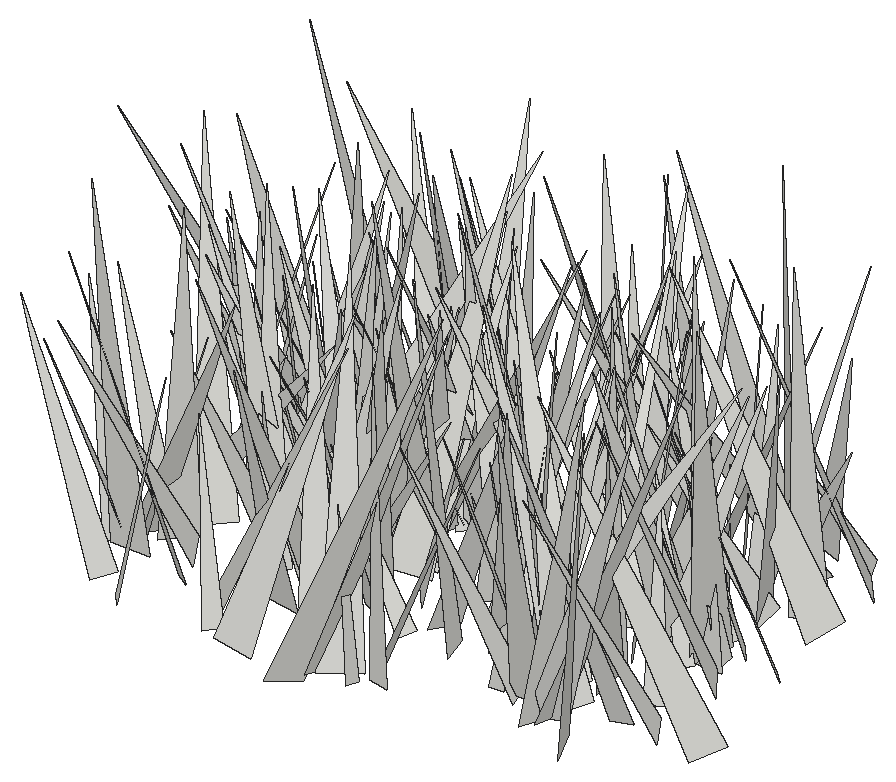
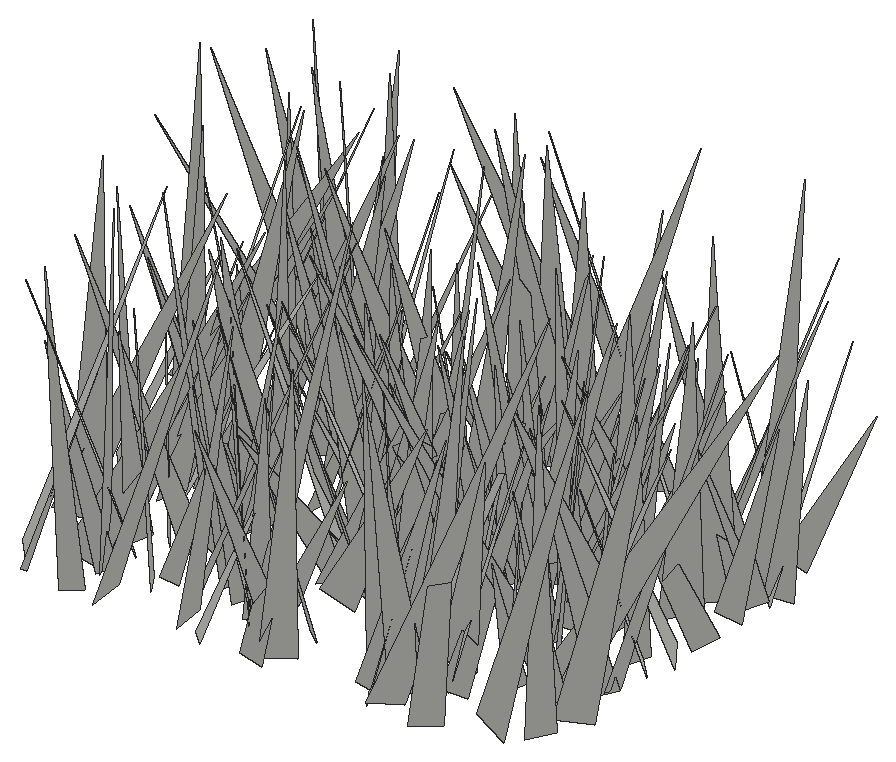
# SketchUp Ruby script. Lengths in inches.
U = 1.inch
M = Sketchup.active_model
def pt(a) = Geom::Point3d.new(a.map { |v| v * U })
def face(e, loops, mat)
  f = e.add_face(loops[0].map { |a| pt(a) })
  loops[1..].each { |l| e.add_face(l.map { |a| pt(a) }).erase! }
  f.material = f.back_material = mat if mat
  f
end
# faces: each face lists its corners as indices into pts; further lists are holes
def faces(e, pts, list, mat = nil) = list.each { |f| face(e, (f[0].is_a?(Array) ? f : [f]).map { |l| l.map { |i| pts[i] } }, mat) }
# xy, xz, yz: faces in a plane at the given z, y or x. An outline is a flat list of corners, or four numbers for a rectangle; further outlines are holes
def ring(l) = l.size == 4 ? [[l[0], l[1]], [l[2], l[1]], [l[2], l[3]], [l[0], l[3]]] : l.each_slice(2).to_a
def flat(e, list, mat, &to3) = list.each { |f| face(e, (f[0].is_a?(Array) ? f : [f]).map { |l| ring(l).map { |u, v| to3.(u, v) } }, mat) }
def xy(e, z, list, mat = nil) = flat(e, list, mat) { |x, y| [x, y, z] }
def xz(e, y, list, mat = nil) = flat(e, list, mat) { |x, z| [x, y, z] }
def yz(e, x, list, mat = nil) = flat(e, list, mat) { |y, z| [x, y, z] }
def lines(e, pts, list) = list.each { |a, b| e.add_line(pt(pts[a]), pt(pts[b])) }
# prism: a flat outline (further loops are holes) pulled along v
def prism(e, loops, v, mat = nil)
  f = face(e, loops, mat); d = Geom::Vector3d.new(v.map { |x| x * U })
  f.pushpull(f.normal.samedirection?(d) ? d.length : -d.length)
end
def box(e, o, s, mat = nil) = prism(e, [[o, [o[0] + s[0], o[1], o[2]], [o[0] + s[0], o[1] + s[1], o[2]], [o[0], o[1] + s[1], o[2]]]], [0, 0, s[2]], mat)
def at(x, y, z, deg = 0) = Geom::Transformation.translation(pt([x, y, z])) * Geom::Transformation.rotation(ORIGIN, Z_AXIS, deg.degrees)
def axes(o, x, y, z) = Geom::Transformation.new([*x, 0, *y, 0, *z, 0, *pt(o).to_a, 1])
def part(name) = M.definitions.add(name)
# library, detail: a bought-in or finely detailed component or shape, given as its bounding box
def library(name, o, s) = part(name).tap { |d| box(d.entities, o, s) }
def detail(e, o, s) = box(e.add_group.entities, o, s)
def put(e, d, t, mat = nil) = e.add_instance(d, t).tap { |i| i.material = mat if mat }
def group(e, t, mat = nil) = e.add_group.tap { |g| g.transformation = t; g.material = mat if mat }.entities
root = M.entities
c1 = part("fur_instance\#9")
p = [[0.8125,0,1.79],[0.67,-0.02,1.48],[0,-0.11,0],[0,0.11,0]]
faces(c1.entities,p,[[0,1,2,3]])
put(root,c1,axes([75.82,233.1,-27.1],[7.81962,-2.04899,1.63917],[-2.46618,-7.49875,2.3913],[-0.8962,2.75717,7.72182]))
put(root,c1,axes([86.82,235.52,-27.1],[6.37942,2.61315,2.43113],[3.05762,-6.56979,-0.96169],[-1.84118,-1.85616,6.82648]))
put(root,c1,axes([67.4,233.97,-27.1],[3.19373,2.97376,0.94617],[2.91746,-3.32577,0.60507],[-1.10768,-0.18543,4.3217]))
put(root,c1,axes([71.48,234.4375,-27.1],[-3.55756,1.9012,0.49829],[1.88183,3.59228,-0.2708],[0.56709,0.00632,4.02461]))
put(root,c1,axes([72.91,233.79,-27.1],[-0.40245,7.17423,1.83924],[7.10701,0.89237,-1.92572],[2.08393,-1.65784,6.92265]))
put(root,c1,axes([70.46,235.91,-27.1],[6.41393,4.45568,0.74677],[4.39818,-5.86174,-2.80093],[1.0328,-2.70854,7.29015]))
put(root,c1,axes([83.7,237.41,-27.1],[0.50064,-7.21064,0.91051],[-7.21991,-0.3887,0.89157],[0.83387,0.96363,7.17281]))
put(root,c1,axes([77.92,234.46,-27.1],[-4.02809,-0.22088,0.67447],[-0.39433,3.92835,-1.06856],[0.59008,1.11738,3.89005]))
put(root,c1,axes([72.41,237.38,-27.1],[-0.34138,-6.1128,0.75859],[-6.1403,0.39794,0.44341],[0.48829,0.7305,6.10625]))
put(root,c1,axes([67.4,238.57,-27.1],[-5.6995,-3.45113,0.56108],[-3.05969,5.44221,2.39374],[1.69215,-1.78365,6.21808]))
put(root,c1,axes([74.41,237.6875,-27.1],[-0.98604,-7.77609,1.14314],[-7.75331,0.77346,-1.42635],[-1.28859,1.29646,7.70749]))
put(root,c1,axes([78.7,234.97,-27.1],[2.01081,5.29668,2.07869],[5.40677,-2.46554,1.0522],[-1.77275,-1.51176,5.56697]))
put(root,c1,axes([64.83,237.87,-27.1],[-3.71629,-3.62879,0.54604],[-3.4741,3.72939,1.13989],[1.18191,-0.44788,5.0675]))
put(root,c1,axes([65.96,235.05,-27.1],[-1.87407,5.07403,0.37598],[4.58214,1.50899,2.47512],[-2.21159,-1.17322,4.80954]))
put(root,c1,axes([83.11,237.68,-27.1],[-5.60277,-1.40853,0.55452],[-1.25772,5.51462,1.29985],[0.84237,-1.13469,5.62898]))
put(root,c1,axes([88.72,238.66,-27.1],[-5.31145,-3.30369,0.30508],[-3.10318,5.15062,1.7494],[1.17379,-1.33255,6.00546]))
put(root,c1,axes([76.02,234.85,-27.1],[-5.00326,5.02156,1.24961],[5.08502,5.09325,-0.10752],[0.95924,-0.80806,7.08781]))
put(root,c1,axes([65.47,237.18,-27.1],[-0.06707,-7.91469,2.47451],[-8.29222,0.04381,-0.08466],[-0.06773,2.47503,7.91452]))
put(root,c1,axes([76.33,234.38,-27.1],[6.99612,0.8962,1.32294],[0.53893,-6.91662,1.83548],[-1.5043,1.69005,6.81028]))
put(root,c1,axes([77.11,234.78,-27.1],[-4.81371,6.17541,1.55135],[6.27572,4.93015,-0.15223],[1.07597,-1.1279,7.82843]))
put(root,c1,axes([68.33,236.62,-27.1],[-4.54723,-4.75664,0.92618],[-4.80738,4.26788,-1.68375],[-0.61038,1.82216,6.36144]))
put(root,c1,axes([85.05,236.82,-27.1],[5.41416,-4.66063,0.97473],[-4.76032,-5.26587,1.26282],[0.1044,1.59183,7.03135]))
put(root,c1,axes([84.84,236.43,-27.1],[6.67765,-1.57713,2.05629],[-1.75682,-6.93326,0.38749],[-1.90506,0.86558,6.85042]))
put(root,c1,axes([81.29,239.26,-27.1],[1.38948,-7.3294,0.52561],[-7.22169,-1.26322,1.47599],[1.35779,0.7818,7.31247]))
put(root,c1,axes([82.22,239.42,-27.1],[-4.28945,-4.51982,0.83876],[-4.25056,4.33652,1.63064],[1.75072,-0.54543,6.01408]))
put(root,c1,axes([74.53,236.67,-27.1],[-0.74897,7.24815,2.93985],[7.55595,1.43371,-1.60981],[2.0214,-2.6736,7.1067]))
put(root,c1,axes([87.3,238.3,-27.1],[-2.01567,-6.30283,1.43527],[-6.28052,1.55369,-1.99742],[-1.52993,1.92587,6.30864]))
put(root,c1,axes([75.15,239.1,-27.1],[-2.33347,-4.94017,0.88075],[-4.99474,2.38012,0.11709],[0.48332,0.74554,5.4623]))
put(root,c1,axes([64.7,237.41,-27.1],[-2.06507,4.56305,1.47225],[4.79287,1.92061,0.77009],[-0.13147,-1.65628,4.94903]))
put(root,c1,axes([85.13,236.9,-27.1],[7.79072,-0.23447,0.87822],[-0.35324,-7.76347,1.06082],[-0.83754,1.09323,7.72172]))
put(root,c1,axes([72.3125,239.3125,-27.1],[-4.28655,1.17606,1.86698],[1.8295,4.17484,1.57066],[1.23356,-2.10497,4.15821]))
put(root,c1,axes([74.13,240.15,-27.1],[5.44226,-5.9088,0.26751],[-5.91243,-5.44486,0.01623],[-0.16928,0.20777,8.03317]))
put(root,c1,axes([91.21,238.4,-27.1],[-4.16636,5.9481,1.52453],[5.74666,3.12806,3.50054],[-2.16332,-3.14611,6.36276]))
put(root,c1,axes([65.1,238.51,-27.1],[5.86888,-2.59714,0.14419],[-2.59865,-5.83866,0.60558],[0.11385,0.61201,6.38922]))
put(root,c1,axes([85.16,240.3125,-27.1],[6.59264,-0.88288,1.14982],[-0.53637,-6.4595,-1.88457],[-1.3468,-1.74924,6.37893]))
put(root,c1,axes([85.06,237.48,-27.1],[-4.32916,0.66549,1.27706],[0.40908,4.44763,-0.93094],[1.38073,0.76884,4.27993]))
put(root,c1,axes([66.33,238.95,-27.1],[-4.86484,4.13925,3.64162],[4.78109,5.5858,0.03796],[2.74517,-2.39309,6.38738]))
put(root,c1,axes([84.28,238.23,-27.1],[-5.98871,-2.33617,1.80164],[-2.60473,6.10133,-0.74665],[1.38529,1.37273,6.38474]))
put(root,c1,axes([77.84,236.35,-27.1],[3.89032,1.8987,0.46131],[1.51623,-3.58179,1.95558],[-1.23244,1.58688,3.86204]))
put(root,c1,axes([85.3125,237.98,-27.1],[-7.32829,2.58062,0.59876],[2.60966,7.33524,0.32553],[0.45582,-0.50666,7.76257]))
put(root,c1,axes([82.47,239.13,-27.1],[5.33637,4.77614,2.80857],[5.34994,-5.45601,-0.88678],[-1.44141,-2.56842,7.10647]))
put(root,c1,axes([79.25,238.71,-27.1],[-6.68963,-2.36331,2.10659],[-2.62997,6.88987,-0.62215],[1.76244,1.31094,7.06748]))
put(root,c1,axes([89.59,239.7,-27.1],[-6.11827,1.22354,0.04324],[1.20265,5.96505,1.37981],[-0.22923,-1.36132,6.08493]))
put(root,c1,axes([77.21,238.49,-27.1],[-1.66623,3.3763,0.05798],[2.90925,1.40249,1.93607],[-1.71436,-0.9015,3.22914]))
put(root,c1,axes([65.49,237.81,-27.1],[3.79033,1.52401,0.8214],[1.29616,-3.80865,1.0854],[-1.14773,0.73179,3.93842]))
put(root,c1,axes([81.27,239.93,-27.1],[-2.39364,-3.13142,1.17859],[-3.27618,2.48779,-0.04385],[0.67935,0.9641,3.94124]))
put(root,c1,axes([68.75,241.16,-27.1],[0.69444,-4.60057,1.02449],[-4.36557,-1.0182,-1.61314],[-1.77671,0.70364,4.36409]))
put(root,c1,axes([82.21,237.4,-27.1],[2.45384,5.3856,0.3895],[5.06414,-2.44383,1.88676],[-1.87372,0.44803,5.60947]))
put(root,c1,axes([83.4375,240.07,-27.1],[-3.37227,-0.8607,0.92289],[-0.91034,3.4828,-0.07828],[0.87397,0.30665,3.4795]))
put(root,c1,axes([88.16,242.69,-27.1],[-5.39374,-4.42373,0.73063],[-4.15874,5.36317,1.77113],[1.67573,-0.92879,6.74722]))
put(root,c1,axes([75.81,241.04,-27.1],[3.73133,2.74864,1.27928],[3.02044,-3.19509,-1.94493],[0.26177,-2.31318,4.20655]))
put(root,c1,axes([65.27,239.65,-27.1],[-1.60239,4.56784,1.22355],[4.62571,1.24567,1.40748],[-0.98238,-1.58525,4.63161]))
put(root,c1,axes([69.11,241.01,-27.1],[3.4639,-0.21189,1.20284],[0.06017,-3.58323,-0.80448],[-1.21988,-0.7784,3.37584]))
put(root,c1,axes([70.13,240.19,-27.1],[-6.35948,3.06032,1.72749],[3.24757,6.48259,0.47123],[1.34279,-1.18457,7.04176]))
put(root,c1,axes([82.43,239.02,-27.1],[3.56611,7.00423,0.23479],[6.50816,-3.2121,-3.02618],[2.59966,-1.56674,7.25387]))
put(root,c1,axes([87.46,240.03,-27.1],[-1.55614,3.71904,0.91385],[3.82438,1.56093,0.15988],[0.20123,-0.90564,4.0283]))
put(root,c1,axes([70.16,240.22,-27.1],[-2.19401,4.08598,0.64459],[3.98986,1.89782,1.55038],[-1.09165,-1.27572,4.37096]))
put(root,c1,axes([73.15,240.28,-27.1],[4.12414,-1.44643,0.07491],[-1.4095,-3.95608,1.21201],[0.33327,1.1677,4.19901]))
put(root,c1,axes([84,239.27,-27.1],[-6.13421,5.52562,0.24546],[5.52788,6.11218,0.5523],[-0.18784,-0.57446,8.23747]))
put(root,c1,axes([70.47,239.15,-27.1],[-6.55915,2.85076,0.80174],[2.70921,6.56329,-1.17278],[1.19574,0.76707,7.05506]))
put(root,c1,axes([82.21,240.03,-27.1],[-0.35457,5.93898,1.63328],[6.05839,0.63143,-0.98081],[1.11129,-1.54746,5.86815]))
put(root,c1,axes([73.56,242.25,-27.1],[-2.21504,-4.22644,0.02495],[-4.06696,2.12371,-1.31133],[-1.15036,0.62998,4.58799]))
put(root,c1,axes([64.6875,241.69,-27.1],[2.58062,-5.27777,0.62862],[-4.46822,-1.77579,3.43383],[2.87837,1.97518,4.76689]))
put(root,c1,axes([69.66,243.11,-27.1],[6.23542,-1.61716,0.46655],[-1.48447,-6.12774,-1.40019],[-0.79324,-1.24458,6.2877]))
put(root,c1,axes([85.625,243.85,-27.1],[5.45366,-4.66647,1.60556],[-4.21255,-5.64853,-2.10822],[-2.57063,-0.64365,6.86103]))
put(root,c1,axes([70.11,241.64,-27.1],[-5.34119,3.3335,0.99515],[3.47843,5.14626,1.43085],[0.05516,-1.74201,6.13133]))
put(root,c1,axes([79.4375,241.07,-27.1],[2.86437,6.58912,2.04567],[6.83224,-2.40073,-1.83379],[0.96006,-2.57407,6.94682]))
put(root,c1,axes([77.86,239.83,-27.1],[7.57177,-0.43303,1.80554],[-0.88332,-7.50835,1.90355],[-1.63317,2.05334,7.34137]))
put(root,c1,axes([81.09,240.08,-27.1],[-3.67286,3.55796,0.5072],[3.52102,3.70767,-0.51167],[0.72023,0.01818,5.08794]))
put(root,c1,axes([74.72,243.12,-27.1],[-1.19832,-8.06423,2.00487],[-8.30399,1.23724,0.01324],[0.30817,1.98109,8.15276]))
put(root,c1,axes([78.06,242.37,-27.1],[3.7544,-3.60472,1.46029],[-3.77286,-3.86843,0.15082],[-0.94444,1.12393,5.20257]))
put(root,c1,axes([84.68,241.25,-27.1],[1.78909,6.44129,2.50482],[6.73985,-2.19865,0.83993],[-1.52927,-2.15428,6.63216]))
put(root,c1,axes([72.03,242.41,-27.1],[-5.02266,3.34128,1.54054],[3.64584,4.87057,1.32283],[0.49523,-1.96924,5.88569]))
put(root,c1,axes([69.45,243.86,-27.1],[3.15853,-4.87453,2.05329],[-4.28659,-3.76007,-2.33247],[-3.09874,0.23284,5.31949]))
put(root,c1,axes([66.7,240.58,-27.1],[-6.24341,4.5177,1.05822],[4.50521,6.32678,-0.4296],[1.11019,-0.26807,7.69449]))
put(root,c1,axes([69.52,242.93,-27.1],[-3.89073,-3.2521,0.98713],[-3.3181,3.95947,-0.03367],[0.73538,0.65937,5.07078]))
put(root,c1,axes([86.81,244.1,-27.1],[7.55718,-3.05255,1.8054],[-2.7949,-7.74218,-1.39129],[-2.18313,-0.65505,8.03077]))
put(root,c1,axes([72.9,242.14,-27.1],[4.30722,-1.10997,0.82887],[-1.21703,-4.32511,0.53238],[-0.66174,0.72977,4.41597]))
put(root,c1,axes([70.14,242.96,-27.1],[-7.66892,-1.90839,0.15613],[-1.91216,7.66661,-0.21311],[0.09999,0.24454,7.89993]))
put(root,c1,axes([66.61,243.5,-27.1],[-5.67591,-0.59927,2.29984],[-0.30227,6.08824,0.84044],[2.35734,-0.66225,5.64524]))
put(root,c1,axes([81.92,242.72,-27.1],[-5.15429,0.32159,0.0951],[0.32057,5.15491,-0.05731],[0.09848,0.05128,5.164]))
put(root,c1,axes([80.93,243.25,-27.1],[-7.3033,-3.33888,1.09507],[-3.45877,7.27632,-0.88176],[0.61989,1.26191,7.98178]))
put(root,c1,axes([69.2,244.77,-27.1],[6.14406,2.36607,3.59044],[3.36505,-6.54408,-1.44586],[-2.67694,-2.79567,6.42319]))
put(root,c1,axes([73.43,245.12,-27.1],[5.23311,-3.59302,0.50013],[-3.53385,-5.24745,-0.7222],[-0.81967,-0.31597,6.30664]))
put(root,c1,axes([71.98,241.91,-27.1],[-5.31881,4.24046,0.31909],[4.24772,5.322,0.07866],[0.20039,-0.26047,6.80184]))
put(root,c1,axes([72.93,240.42,-27.1],[1.87355,6.48838,0.26131],[6.01197,-1.83596,2.48253],[-2.45429,0.45575,6.28063]))
put(root,c1,axes([87.48,244.02,-27.1],[-3.67755,-0.2078,1.11626],[-0.0694,3.8179,0.48208],[1.13331,-0.4405,3.65173]))
put(root,c1,axes([71.16,242.97,-27.1],[1.59622,5.71911,2.00108],[6.0184,-1.73595,0.16062],[-0.70101,-1.88115,5.93551]))
put(root,c1,axes([84.43,242.48,-27.1],[5.20843,4.28763,1.83578],[4.29945,-5.48037,0.60158],[-1.80791,-0.68076,6.71935]))
put(root,c1,axes([89.64,244.41,-27.1],[-3.75562,-3.58045,0.3486],[-3.58145,3.67402,-0.84892],[-0.33818,0.85312,5.11895]))
put(root,c1,axes([65.1875,246.42,-27.1],[-6.16239,-2.08969,1.53365],[-1.42213,6.03269,2.50561],[2.16712,-1.98337,6.00531]))
put(root,c1,axes([79.35,242.23,-27.1],[3.38601,2.0667,0.33408],[1.88033,-3.28152,1.24252],[-0.92044,0.89903,3.76728]))
put(root,c1,axes([86.52,242.93,-27.1],[-0.98772,3.5916,0.11089],[3.35733,0.88143,1.35606],[-1.28071,-0.45933,3.46934]))
put(root,c1,axes([74.43,242.02,-27.1],[-3.17908,7.18759,1.82609],[7.05927,3.54175,-1.65087],[2.27218,-0.9472,7.68392]))
put(root,c1,axes([87.15,243.37,-27.1],[1.25442,7.48082,2.76942],[7.81491,-1.71475,1.09211],[-1.59984,-2.51056,7.50623]))
put(root,c1,axes([72.58,243.89,-27.1],[4.97792,-1.2009,1.19397],[-1.36113,-5.04298,0.6026],[-1.0075,0.87956,5.08515]))
put(root,c1,axes([85.42,243.25,-27.1],[0.44188,5.84269,1.52194],[5.83939,-0.02571,-1.59672],[1.53457,-1.58458,5.63763]))
put(root,c1,axes([74.9,246.1875,-27.1],[1.62052,-5.44249,0.65001],[-5.43307,-1.68456,-0.55967],[-0.72449,0.45919,5.65098]))
put(root,c1,axes([87.62,245.02,-27.1],[-4.41159,-3.54695,0.73212],[-3.61607,4.3782,-0.57829],[0.20221,0.91078,5.63104]))
put(root,c1,axes([73.36,242.16,-27.1],[1.09357,6.43106,0.77169],[6.11568,-1.28298,2.02542],[-2.13365,-0.38127,6.20097]))
put(root,c1,axes([72.23,245.85,-27.1],[-3.11173,-3.4795,0.92655],[-3.33661,3.24675,0.98692],[1.3537,0.0043,4.56244]))
put(root,c1,axes([65.85,244.22,-27.1],[-4.75498,1.70819,1.94206],[1.76287,5.11453,-0.18234],[1.89256,-0.47231,5.04921]))
put(root,c1,axes([73.33,246.44,-27.1],[-3.18461,-4.17271,0.10236],[-4.17132,3.18622,0.10881],[0.1486,0.01532,5.24799]))
put(root,c1,axes([75.9,246.87,-27.1],[-1.54524,-6.7658,0.51217],[-6.71547,1.44992,-1.10738],[-0.96994,0.74015,6.85109]))
put(root,c1,axes([77.31,245.02,-27.1],[6.16664,-2.56617,1.31423],[-2.70082,-6.22755,0.51287],[-1.00896,0.98602,6.65955]))
put(root,c1,axes([69.11,245.34,-27.1],[7.358,-0.55238,1.16955],[-0.51092,-7.44716,-0.30295],[-1.18825,-0.21839,7.37248]))
put(root,c1,axes([73.91,243.53,-27.1],[7.28902,-0.71217,0.57332],[-0.83779,-7.04721,1.89755],[-0.36604,1.94818,7.07364]))
put(root,c1,axes([67.05,247.09,-27.1],[-1.39061,-8.04384,0.83594],[-7.45661,0.94696,-3.29214],[-3.13068,1.31752,7.46987]))
put(root,c1,axes([74.43,242.78,-27.1],[-1.14169,6.19263,0.48775],[6.13199,1.20279,-0.91762],[0.99261,-0.30768,6.22978]))
put(root,c1,axes([67.7,246.54,-27.1],[-3.39488,-3.98848,1.56761],[-3.7052,3.73666,1.48306],[2.15333,0.14147,5.02331]))
put(root,c1,axes([66.82,245.58,-27.1],[-2.76326,-3.0585,1.38467],[-3.15346,2.97986,0.28892],[1.15213,0.82059,4.11176]))
put(root,c1,axes([86.87,243.74,-27.1],[-6.97142,-3.26118,0.0354],[-2.96258,6.29742,-3.28677],[-1.3637,2.99072,6.9594]))
put(root,c1,axes([78.18,246.59,-27.1],[-6.07615,0.58264,0.90457],[0.83184,5.83413,1.82981],[0.68247,-1.92372,5.8233]))
put(root,c1,axes([77.59,244,-27.1],[-3.01404,5.97197,0.86388],[5.95256,2.78442,1.51964],[-0.98886,-1.44144,6.51457]))
put(root,c1,axes([65,243,-27.1],[5.18703,3.91751,0.7095],[3.72248,-5.18551,1.41748],[-1.41191,0.72053,6.34373]))
put(root,c1,axes([74.58,246.28,-27.1],[2.81734,-6.20209,1.85033],[-6.41792,-2.93797,-0.07572],[-0.83667,1.65211,6.81158]))
put(root,c1,axes([77.36,246.38,-27.1],[-4.25466,-1.2014,1.34721],[-0.93808,4.41863,0.97784],[1.54219,-0.62673,4.31153]))
put(root,c1,axes([76.05,245.7,-27.1],[-1.30466,-3.28465,1.2487],[-3.51229,1.2605,-0.354],[0.10971,1.29326,3.5165]))
put(root,c1,axes([77.03,244.09,-27.1],[4.58247,4.01128,0.43645],[4.00699,-4.60163,0.22113],[-0.47421,-0.12046,6.08609]))
put(root,c1,axes([79.41,243.99,-27.1],[-0.73079,4.32054,0.1844],[4.30671,0.74406,-0.36572],[0.39156,-0.12013,4.36662]))
put(root,c1,axes([86.65,247.64,-27.1],[-4.86866,0.51762,1.11395],[0.97098,4.41082,2.19421],[0.75234,-2.34296,4.3769]))
put(root,c1,axes([78.57,245.125,-27.1],[5.68273,3.19615,0.64935],[3.24559,-5.67036,-0.49352],[-0.32122,-0.74969,6.50117]))
put(root,c1,axes([82.98,245.58,-27.1],[2.29321,-4.71361,1.70331],[-4.8602,-1.63403,2.02152],[1.22385,2.34308,4.83635]))
put(root,c1,axes([67.81,243.09,-27.1],[-5.19171,3.73852,1.55221],[3.028,5.26206,-2.54592],[2.68647,1.29382,5.8693]))
put(root,c1,axes([86.6,245.11,-27.1],[-5.80582,1.67481,0.45332],[1.66732,5.82342,-0.1609],[0.48013,0.02943,6.04042]))
put(root,c1,axes([75.09,245.7,-27.1],[-3.69691,-1.68274,0.52652],[-1.75981,3.59718,-0.85985],[0.10916,1.00233,3.96981]))
put(root,c1,axes([65.32,244.39,-27.1],[3.04107,3.48011,0.59696],[3.3547,-3.09349,0.94446],[-1.10161,0.1866,4.52408]))
put(root,c1,axes([65.24,246.77,-27.1],[2.87453,-4.20489,0.68169],[-4.14129,-2.56592,1.63539],[0.99777,1.46412,4.82385]))
put(root,c1,axes([86.32,247.76,-27.1],[6.10646,0.88523,1.50787],[1.27518,-6.00248,-1.64024],[-1.19633,-1.87958,5.94829]))
put(root,c1,axes([82.58,245.01,-27.1],[-5.70861,3.53079,2.01517],[3.32922,6.05385,-1.17592],[2.33318,0.00055,6.60847]))
put(root,c1,axes([68.99,247.32,-27.1],[-4.42725,-2.60663,1.07476],[-2.66002,4.52485,0.01676],[0.93485,0.53053,5.13759]))
put(root,c1,axes([74.09,245.88,-27.1],[-3.60805,2.068,0.36238],[2.05277,3.62596,-0.25393],[0.44056,0.04128,4.15092]))
put(root,c1,axes([66.03,248.58,-27.1],[-3.26059,-4.43586,0.10579],[-4.43536,3.26207,0.0775],[0.12511,0.03932,5.50476]))
put(root,c1,axes([82.9,245.93,-27.1],[-6.0397,-1.24718,1.08354],[-1.47294,5.92489,-1.39057],[0.74831,1.59618,6.00831]))
put(root,c1,axes([69.53,250.18,-27.1],[4.70734,-3.12135,0.14145],[-2.64852,-4.12178,-2.81392],[-1.65776,-2.27815,4.89732]))
put(root,c1,axes([72.9,244.54,-27.1],[-1.71935,6.00909,0.23442],[5.94835,1.73522,-0.85232],[0.8839,0.01135,6.19184]))
put(root,c1,axes([88.93,248.03,-27.1],[-7.28796,2.50197,0.93453],[2.66483,6.99355,2.0583],[0.17855,-2.25345,7.42547]))
put(root,c1,axes([82.76,243.8,-27.1],[-4.41357,6.91206,0.00056],[6.86097,4.38103,-0.99489],[0.83882,0.53496,8.14041]))
put(root,c1,axes([82.66,247.55,-27.1],[-2.78435,-5.66723,3.39056],[-5.97834,3.72634,1.319],[2.80584,2.3158,6.17497]))
put(root,c1,axes([75.77,247.13,-27.1],[4.35224,4.23695,0.82253],[4.28263,-4.09432,-1.57033],[0.53605,-1.68972,5.86752]))
put(root,c1,axes([64.83,249.1,-27.1],[4.91943,-4.73173,2.30235],[-4.40019,-5.42749,-1.75256],[-2.8859,0.2095,6.59686]))
put(root,c1,axes([86.2,250.79,-27.1],[2.18391,-6.70079,0.42323],[-6.08063,-2.16263,-2.86325],[-2.84706,-0.52116,6.43986]))
put(root,c1,axes([84.6,247.8125,-27.1],[2.87799,2.64757,1.74089],[2.94858,-3.09885,-0.16173],[-1.16026,-1.30792,3.90721]))
put(root,c1,axes([80.87,251.1875,-27.1],[-6.78403,-3.28205,0.63683],[-2.89291,6.48484,2.60352],[1.67585,-2.09175,7.07224]))
put(root,c1,axes([87.93,248.39,-27.1],[1.68119,-6.78383,2.85706],[-7.30642,-1.89388,-0.19753],[-0.89411,2.72073,6.98625]))
put(root,c1,axes([83.46,247.74,-27.1],[6.47298,0.85818,0.33872],[0.84258,-6.4766,0.30739],[-0.37587,0.26066,6.52238]))
put(root,c1,axes([67.67,249.43,-27.1],[3.15596,1.30372,1.61225],[1.82364,-3.14251,-1.02861],[-0.98659,-1.6383,3.25603]))
put(root,c1,axes([80.8125,249.11,-27.1],[3.7872,-0.0255,0.26622],[0.02172,-3.73751,-0.66706],[-0.26655,-0.66693,3.72808]))
put(root,c1,axes([70.03,249.9,-27.1],[-3.79874,-3.55526,0.6962],[-3.51199,3.8615,0.55657],[0.88909,0.06302,5.17306]))
put(root,c1,axes([79.05,245.22,-27.1],[-4.90566,2.32822,0.51514],[1.6552,4.17303,-3.098],[1.71648,2.62995,4.45965]))
put(root,c1,axes([68.17,246.625,-27.1],[0.84349,7.5995,0.98427],[7.14395,-0.42161,-2.86687],[2.77222,-1.22577,7.08837]))
put(root,c1,axes([82.73,250.12,-27.1],[0.53786,-3.60504,0.14249],[-3.55289,-0.5543,-0.6129],[-0.62738,0.04841,3.59304]))
put(root,c1,axes([78.45,248.54,-27.1],[-1.80359,3.13263,0.44398],[3.00697,1.53819,1.36218],[-0.98418,-1.04117,3.34825]))
put(root,c1,axes([73.66,248.06,-27.1],[0.00503,4.167,0.7042],[4.17874,-0.11,0.62111],[-0.63075,-0.69557,4.12045]))
put(root,c1,axes([72.98,249.04,-27.1],[4.34542,2.75412,2.00138],[2.98226,-4.64462,-0.0836],[-1.6422,-1.14703,5.14401]))
put(root,c1,axes([77.11,247.42,-27.1],[-1.95645,6.57203,0.15793],[5.85701,1.66776,3.15567],[-2.98529,-1.03499,6.08778]))
put(root,c1,axes([79.6875,249.49,-27.1],[5.0608,-1.8582,0.79428],[-1.91101,-5.09708,0.2516],[-0.65714,0.51221,5.38529]))
put(root,c1,axes([78.59,250.46,-27.1],[4.23217,0.79223,1.75299],[1.35483,-4.23497,-1.35698],[-1.36567,-1.74623,4.08626]))
put(root,c1,axes([69.9375,251.125,-27.1],[-3.5221,-6.63629,1.77015],[-6.5539,3.84233,1.36448],[2.0543,0.8804,7.38808]))
put(root,c1,axes([66.11,248.4,-27.1],[0.58745,4.61701,1.14714],[4.75417,-0.52722,-0.31264],[0.17496,-1.17604,4.64372]))
put(root,c1,axes([88.25,251.58,-27.1],[-5.65228,-5.31186,0.60473],[-5.29476,5.68375,0.43618],[0.73959,0.09466,7.74428]))
put(root,c1,axes([85.47,248.43,-27.1],[-4.49774,2.41965,1.22715],[2.26445,4.65664,-0.88215],[1.49428,0.22634,5.03052]))
put(root,c1,axes([65.13,250.64,-27.1],[5.79339,-2.08626,1.56673],[-1.97661,-6.00002,-0.68061],[-1.70297,-0.13319,6.11985]))
put(root,c1,axes([76.8,252.8,-27.1],[-3.41876,-7.6362,0.72671],[-7.48826,3.49493,1.49637],[1.66304,0.03883,8.23167]))
put(root,c1,axes([84.99,250.88,-27.1],[1.43751,-4.12245,0.23292],[-3.7226,-1.18725,1.96162],[1.78636,0.84328,3.90039]))
put(root,c1,axes([71,252.29,-27.1],[-7.92224,1.63819,2.17065],[2.33717,7.51957,2.85498],[1.39032,-3.306,7.56932]))
put(root,c1,axes([68.85,252.64,-27.1],[6.56004,-2.8558,0.90961],[-2.50702,-6.42798,-2.10074],[-1.6425,-1.59457,6.83935]))
put(root,c1,axes([68.02,248.45,-27.1],[-3.33951,2.40161,0.05247],[2.31618,3.24301,-1.02031],[0.63702,0.79874,3.98485]))
put(root,c1,axes([72.96,250.1,-27.1],[5.47635,-0.94494,2.24683],[-1.1073,-5.8869,0.22307],[-2.17142,0.61884,5.55279]))
put(root,c1,axes([76.0625,250.09,-27.1],[4.67492,4.49227,1.13099],[4.6277,-4.45606,-1.42912],[0.20972,-1.8104,6.324]))
put(root,c1,axes([70.71,248.45,-27.1],[-2.20757,6.36235,0.08993],[6.1827,2.12231,1.62203],[-1.50393,-0.61421,6.5362]))
put(root,c1,axes([83.06,250.67,-27.1],[4.36466,2.86173,1.95624],[3.18404,-4.55325,-0.44325],[-1.3705,-1.46462,5.20032]))
put(root,c1,axes([87.36,252.74,-27.1],[-3.37323,-1.69913,0.74168],[-1.13548,3.11072,1.96213],[1.46554,-1.50074,3.22735]))
put(root,c1,axes([85.39,248.9,-27.1],[4.30738,5.01035,0.65824],[4.94004,-4.35705,0.83813],[-1.06435,0.05398,6.55397]))
put(root,c1,axes([66.9375,251.31,-27.1],[-2.69995,-7.06667,2.40673],[-7.39529,2.18224,-1.88876],[-1.01973,2.88442,7.32531]))
put(root,c1,axes([78.63,250.6875,-27.1],[-4.89725,-3.9807,3.26033],[-4.56553,5.43754,-0.21877],[2.37312,2.24631,6.30723]))
put(root,c1,axes([85.51,250.34,-27.1],[-6.98093,-2.98191,2.95578],[-3.56155,7.24267,-1.10492],[2.22346,2.23913,7.51028]))
put(root,c1,axes([78.3,250.51,-27.1],[-1.55203,4.86816,1.43833],[5.0761,1.479,0.47157],[-0.03172,-1.51332,5.08777]))
put(root,c1,axes([78.52,250.49,-27.1],[2.84043,2.51238,0.82611],[2.52394,-2.93724,0.2547],[-0.79009,-0.35083,3.78354]))
put(root,c1,axes([85.09,252.79,-27.1],[0.27487,-5.90315,0.86813],[-5.62576,0.03312,2.00651],[1.98787,0.91,5.55848]))
put(root,c1,axes([79.32,252.72,-27.1],[-2.85386,-2.94003,0.13695],[-2.93623,2.85714,0.14971],[0.2028,-0.00613,4.09462]))
put(root,c1,axes([72.04,251.84,-27.1],[-1.46223,5.38545,2.28823],[5.73287,0.84616,1.67196],[-1.17188,-2.58033,5.32407]))
put(root,c1,axes([83.88,252.34,-27.1],[-7.9003,-1.05971,0.99848],[-1.05239,7.96314,0.1246],[1.0062,0.00826,7.97008]))
put(root,c1,axes([71.79,252.27,-27.1],[-4.56615,-2.82263,0.99228],[-2.92894,4.58662,-0.43101],[0.61084,0.89289,5.35081]))
put(root,c1,axes([80.45,251.85,-27.1],[-6.61174,-0.50833,1.66504],[-0.62205,6.79727,-0.39495],[1.62598,0.53342,6.61948]))
put(root,c1,axes([76.11,252.1,-27.1],[-4.07853,4.6775,2.02917],[4.97181,4.22458,0.25488],[1.13033,-1.70436,6.20068]))
put(root,c1,axes([76.8125,251.05,-27.1],[-1.32926,4.80497,0.97182],[4.66035,1.55098,-1.29408],[1.52094,-0.553,4.81456]))
put(root,c1,axes([70.79,251.1875,-27.1],[-3.43213,5.64571,1.59286],[5.69776,3.64732,-0.65059],[1.39526,-1.00684,6.57497]))
